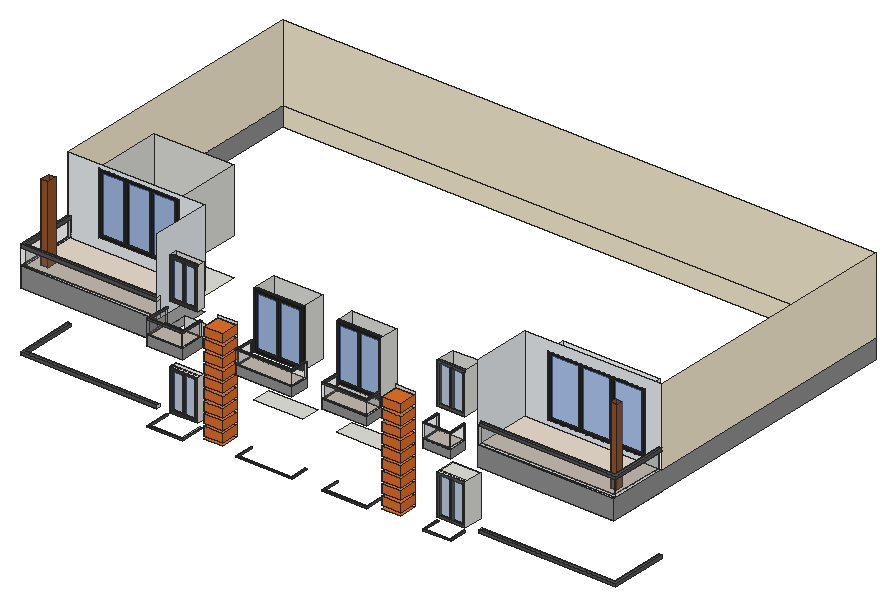
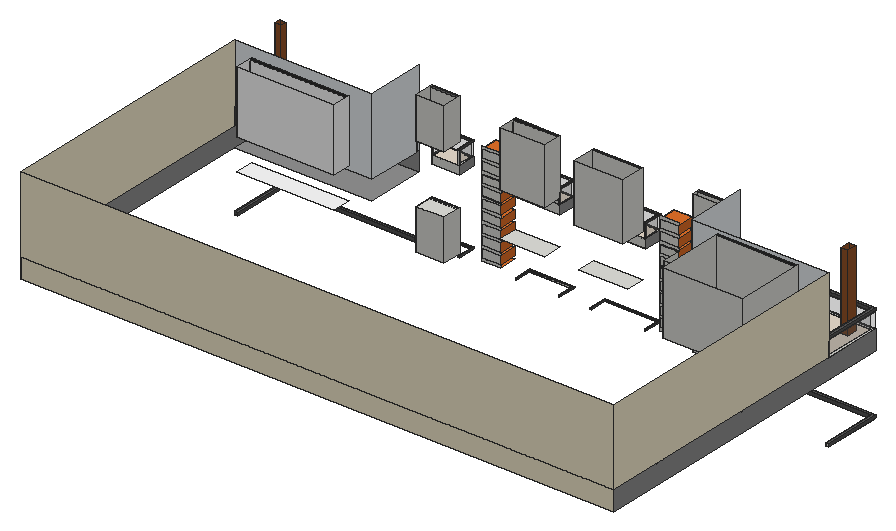
# SketchUp Ruby script. Lengths in inches.
U = 1.inch
M = Sketchup.active_model
def pt(a) = Geom::Point3d.new(a.map { |v| v * U })
def face(e, loops, mat)
  f = e.add_face(loops[0].map { |a| pt(a) })
  loops[1..].each { |l| e.add_face(l.map { |a| pt(a) }).erase! }
  f.material = f.back_material = mat if mat
  f
end
# faces: each face lists its corners as indices into pts; further lists are holes
def faces(e, pts, list, mat = nil) = list.each { |f| face(e, (f[0].is_a?(Array) ? f : [f]).map { |l| l.map { |i| pts[i] } }, mat) }
# xy, xz, yz: faces in a plane at the given z, y or x. An outline is a flat list of corners, or four numbers for a rectangle; further outlines are holes
def ring(l) = l.size == 4 ? [[l[0], l[1]], [l[2], l[1]], [l[2], l[3]], [l[0], l[3]]] : l.each_slice(2).to_a
def flat(e, list, mat, &to3) = list.each { |f| face(e, (f[0].is_a?(Array) ? f : [f]).map { |l| ring(l).map { |u, v| to3.(u, v) } }, mat) }
def xy(e, z, list, mat = nil) = flat(e, list, mat) { |x, y| [x, y, z] }
def xz(e, y, list, mat = nil) = flat(e, list, mat) { |x, z| [x, y, z] }
def yz(e, x, list, mat = nil) = flat(e, list, mat) { |y, z| [x, y, z] }
def lines(e, pts, list) = list.each { |a, b| e.add_line(pt(pts[a]), pt(pts[b])) }
# prism: a flat outline (further loops are holes) pulled along v
def prism(e, loops, v, mat = nil)
  f = face(e, loops, mat); d = Geom::Vector3d.new(v.map { |x| x * U })
  f.pushpull(f.normal.samedirection?(d) ? d.length : -d.length)
end
def box(e, o, s, mat = nil) = prism(e, [[o, [o[0] + s[0], o[1], o[2]], [o[0] + s[0], o[1] + s[1], o[2]], [o[0], o[1] + s[1], o[2]]]], [0, 0, s[2]], mat)
def at(x, y, z, deg = 0) = Geom::Transformation.translation(pt([x, y, z])) * Geom::Transformation.rotation(ORIGIN, Z_AXIS, deg.degrees)
def axes(o, x, y, z) = Geom::Transformation.new([*x, 0, *y, 0, *z, 0, *pt(o).to_a, 1])
def part(name) = M.definitions.add(name)
# library, detail: a bought-in or finely detailed component or shape, given as its bounding box
def library(name, o, s) = part(name).tap { |d| box(d.entities, o, s) }
def detail(e, o, s) = box(e.add_group.entities, o, s)
def put(e, d, t, mat = nil) = e.add_instance(d, t).tap { |i| i.material = mat if mat }
def group(e, t, mat = nil) = e.add_group.tap { |g| g.transformation = t; g.material = mat if mat }.entities
root = M.entities
M.materials.add("Generic").color = [146, 146, 146]
M.materials.add("Generic\#3").color = [226, 112, 41]
M.materials.add("Generic\#4").color = [237, 241, 244]
M.materials.add("Generic\#5").color = [249, 239, 211]
M.materials.add("Generic\#7").color = [232, 220, 205]
M.materials.add("[Color M00]").color = [255, 255, 255]
M.materials.add("[Color M06]").color = [86, 86, 86]
M.materials.add("[Color M07]").color = [58, 58, 58]
M.materials.add("[Color M08]").color = [30, 30, 30]
M.materials.add("[Translucent Glass Blue]").color = [98, 147, 234]
M.materials["[Translucent Glass Blue]"].alpha = 0.27
M.materials.add("[Translucent Glass Blue]1").color = [100, 149, 237]
M.materials["[Translucent Glass Blue]1"].alpha = 0.5
M.materials.add("[Translucent Glass Gray]").color = [119, 119, 119]
M.materials["[Translucent Glass Gray]"].alpha = 0.16
M.materials.add("[Wood Cherry Original]").color = [150, 85, 41]
M.materials.add("[Wood Cherry Original]1").color = [152, 86, 42]
c1 = part("Group\#1")
xy(c1.entities,0,[[0,0,60.75,6]],"[Color M07]")
xy(c1.entities,5.51,[[5.51,0,27.62,3],[33.13,0,55.24,3]],"[Color M07]")
xy(c1.entities,84.62,[[5.51,0,27.62,3],[33.13,0,55.24,3]])
xy(c1.entities,90.125,[[0,0,60.75,6]],"[Color M07]")
xz(c1.entities,0,[[[0,0,60.75,90.125],[5.51,5.51,27.62,84.62],[33.13,5.51,55.24,84.62]]],"[Color M07]")
xz(c1.entities,3,[[5.51,5.51,27.62,84.62],[33.13,5.51,55.24,84.62]],"[Translucent Glass Blue]")
xz(c1.entities,6,[[0,0,60.75,90.125]])
yz(c1.entities,0,[[0,0,6,90.125]],"[Color M07]")
yz(c1.entities,5.51,[[0,5.51,3,84.62]],"[Color M07]")
yz(c1.entities,27.62,[[0,5.51,3,84.62]],"[Color M07]")
yz(c1.entities,33.13,[[0,5.51,3,84.62]],"[Color M07]")
yz(c1.entities,55.24,[[0,5.51,3,84.62]],"[Color M07]")
yz(c1.entities,60.75,[[0,0,6,90.125]],"[Color M07]")
c2 = part("Group\#2")
xy(c2.entities,0,[[0,0,60.75,6]],"[Color M06]")
xy(c2.entities,4.875,[[4.875,0,27.9375,3],[32.8125,0,55.875,3]],"[Color M06]")
xy(c2.entities,85.25,[[4.875,0,27.9375,3],[32.8125,0,55.875,3]],"[Color M06]")
xy(c2.entities,90.125,[[0,0,60.75,6]],"[Color M06]")
xz(c2.entities,0,[[[0,0,60.75,90.125],[4.875,4.875,27.9375,85.25],[32.8125,4.875,55.875,85.25]]],"[Color M06]")
xz(c2.entities,3,[[4.875,4.875,27.9375,85.25],[32.8125,4.875,55.875,85.25]],"[Translucent Glass Blue]")
xz(c2.entities,6,[[0,0,60.75,90.125]])
yz(c2.entities,0,[[0,0,6,90.125]],"[Color M06]")
yz(c2.entities,4.875,[[0,4.875,3,85.25]],"[Color M06]")
yz(c2.entities,27.9375,[[0,4.875,3,85.25]],"[Color M06]")
yz(c2.entities,32.8125,[[0,4.875,3,85.25]],"[Color M06]")
yz(c2.entities,55.875,[[0,4.875,3,85.25]],"[Color M06]")
yz(c2.entities,60.75,[[0,0,6,90.125]],"[Color M06]")
c3 = part("Group\#12")
xy(c3.entities,0,[[0,0,212.5625,7]],"[Color M08]")
xy(c3.entities,6.29,[[6.29,0,68.76,4],[75.05,0,137.52,4],[143.8,0,206.27,4]],"[Color M08]")
xy(c3.entities,131.21,[[6.29,0,68.76,4],[75.05,0,137.52,4],[143.8,0,206.27,4]],"[Color M08]")
xy(c3.entities,137.5,[[0,0,212.5625,7]],"[Color M08]")
xz(c3.entities,0,[[0,0,212.5625,6.29],[0,6.29,6.29,131.21],[68.76,6.29,75.05,131.21],[137.52,6.29,143.8,131.21],[206.27,6.29,212.5625,131.21],
  [0,131.21,212.5625,137.5]],"[Color M08]")
xz(c3.entities,4,[[6.29,6.29,68.76,131.21],[75.05,6.29,137.52,131.21],[143.8,6.29,206.27,131.21]],"[Translucent Glass Blue]1")
xz(c3.entities,7,[[0,0,212.5625,137.5]],"[Color M00]")
yz(c3.entities,0,[[0,0,7,137.5]],"[Color M08]")
yz(c3.entities,6.29,[[0,6.29,4,131.21]],"[Color M08]")
yz(c3.entities,68.76,[[0,6.29,4,131.21]],"[Color M08]")
yz(c3.entities,75.05,[[0,6.29,4,131.21]],"[Color M08]")
yz(c3.entities,137.52,[[0,6.29,4,131.21]],"[Color M08]")
yz(c3.entities,143.8,[[0,6.29,4,131.21]],"[Color M08]")
yz(c3.entities,206.27,[[0,6.29,4,131.21]],"[Color M08]")
yz(c3.entities,212.5625,[[0,0,7,137.5]],"[Color M08]")
c4 = part("Group\#10")
xy(c4.entities,0,[[0,0,98.1875,6]],"[Color M08]")
xy(c4.entities,5.79,[[5.79,0,46.2,3],[51.99,0,92.4,3]],"[Color M08]")
xy(c4.entities,117.02,[[5.79,0,46.2,3],[51.99,0,92.4,3]],"[Color M08]")
xy(c4.entities,122.8125,[[0,0,98.1875,6]],"[Color M08]")
xz(c4.entities,0,[[[0,0,98.1875,122.8125],[5.79,5.79,46.2,117.02],[51.99,5.79,92.4,117.02]]],"[Color M08]")
xz(c4.entities,3,[[5.79,5.79,46.2,117.02],[51.99,5.79,92.4,117.02]],"[Translucent Glass Blue]1")
xz(c4.entities,6,[[0,0,98.1875,122.8125]])
yz(c4.entities,0,[[0,0,6,122.8125]],"[Color M08]")
yz(c4.entities,5.79,[[0,5.79,3,117.02]],"[Color M08]")
yz(c4.entities,46.2,[[0,5.79,3,117.02]],"[Color M08]")
yz(c4.entities,51.99,[[0,5.79,3,117.02]],"[Color M08]")
yz(c4.entities,92.4,[[0,5.79,3,117.02]],"[Color M08]")
yz(c4.entities,98.1875,[[0,0,6,122.8125]],"[Color M08]")
c5 = part("Group\#11")
xy(c5.entities,0,[[0,0,175.8125,6]],"[Color M08]")
xy(c5.entities,7.33,[[7.33,0,56.16,3],[63.49,0,112.32,3],[119.65,0,168.48,3]],"[Color M08]")
xy(c5.entities,131.1,[[7.33,0,56.16,3],[63.49,0,112.32,3],[119.65,0,168.48,3]],"[Color M08]")
xy(c5.entities,138.4375,[[0,0,175.8125,6]],"[Color M08]")
xz(c5.entities,0,[[[0,0,175.8125,0,175.8125,131.1,168.48,131.1,168.48,7.33,119.65,7.33,119.65,131.1,175.8125,131.1,175.8125,138.4375,0,138.4375],[7.33,7.33,56.16,131.1],[63.49,7.33,112.32,131.1]]],"[Color M08]")
xz(c5.entities,3,[[7.33,7.33,56.16,131.1],[63.49,7.33,112.32,131.1],[119.65,7.33,168.48,131.1]],"[Translucent Glass Blue]1")
xz(c5.entities,6,[[0,0,175.8125,138.4375]])
yz(c5.entities,0,[[0,0,6,138.4375]],"[Color M08]")
yz(c5.entities,7.33,[[0,7.33,3,131.1]],"[Color M08]")
yz(c5.entities,56.16,[[0,7.33,3,131.1]],"[Color M08]")
yz(c5.entities,63.49,[[0,7.33,3,131.1]],"[Color M08]")
yz(c5.entities,112.32,[[0,7.33,3,131.1]],"[Color M08]")
yz(c5.entities,119.65,[[0,7.33,3,131.1]],"[Color M08]")
yz(c5.entities,168.48,[[0,7.33,3,131.1]],"[Color M08]")
yz(c5.entities,175.8125,[[0,0,6,138.4375]],"[Color M08]")
xy(root,1083.75,[[529.46,261.625,529.46,313.625,532.46,313.625,532.46,264.625,604.09,264.625,604.09,313.625,607.09,313.625,607.09,261.625],[714.9,273.75,838.15,276.75],[903.71,273.75,1001.9,276.75],[1125.09,273.75,1185.84,276.75],[714.9,276.75,717.9,313.625],
  [835.15,276.75,838.15,313.625],[903.71,276.75,906.71,313.625],[998.9,276.75,1001.9,313.625],[1125.09,276.75,1128.09,313.625],[1182.84,276.75,1185.84,313.625]])
xy(root,1086.5,[[529.46,261.625,607.09,261.625,607.09,313.625,604.09,313.625,604.09,264.625,532.46,264.625,532.46,313.625,529.46,313.625]],"[Color M06]")
xy(root,1086.75,[[714.9,273.75,838.15,273.75,838.15,313.625,835.15,313.625,835.15,276.75,717.9,276.75,717.9,313.625,714.9,313.625],[903.71,273.75,1001.9,273.75,1001.9,313.625,998.9,313.625,998.9,276.75,906.71,276.75,906.71,313.625,903.71,313.625],[1125.09,273.75,1185.84,273.75,1185.84,313.625,1182.84,313.625,1182.84,276.75,1128.09,276.75,1128.09,313.625,1125.09,313.625]],"[Color M06]")
xy(root,1089.75,[[209.5,313.625,509.5,320.625],[1213,318.25,1213,325.0625,1506,325.0625,1506,444.3125,1513,444.3125,1513,318.25],[209.5,320.625,216.5,444.3125]])
xy(root,1092.02,[[537.9,313.625,598.65,331.25],[1125.09,313.625,1185.84,356.375]])
xy(root,1094.87,[[643.375,273.75,685.0625,313.625],[1034.5,273.75,1076.1875,313.625]],"Generic\#3")
xy(root,1096.1875,[[1213,318.25,1513,318.25,1513,444.3125,1506,444.3125,1506,325.0625,1213,325.0625]],"[Color M06]")
xy(root,1096.75,[[209.5,313.625,509.5,313.625,509.5,320.625,216.5,320.625,216.5,444.3125,209.5,444.3125]],"[Color M06]")
xy(root,1101.37,[[643.375,273.75,685.0625,313.625],[1034.5,273.75,1076.1875,313.625]],"Generic\#3")
xy(root,1119.37,[[643.375,273.75,685.0625,313.625],[1034.5,273.75,1076.1875,313.625]],"Generic\#3")
xy(root,1125.87,[[643.375,273.75,685.0625,313.625],[1034.5,273.75,1076.1875,313.625]],"Generic\#3")
xy(root,1143.87,[[643.375,273.75,685.0625,313.625],[1034.5,273.75,1076.1875,313.625]],"Generic\#3")
xy(root,1150.37,[[643.375,273.75,685.0625,313.625],[1034.5,273.75,1076.1875,313.625]],"Generic\#3")
xy(root,1168.37,[[643.375,273.75,685.0625,313.625],[1034.5,273.75,1076.1875,313.625]],"Generic\#3")
xy(root,1174.87,[[643.375,273.75,685.0625,313.625],[1034.5,273.75,1076.1875,313.625]],"Generic\#3")
xy(root,1182.05,[[722.84,313.625,830.21,354]])
xy(root,1182.15,[[537.9,313.625,598.65,331.25],[903.71,313.625,1001.9,356.375],[1125.09,313.625,1185.84,356.375]])
xy(root,1192.87,[[643.375,273.75,685.0625,313.625],[1034.5,273.75,1076.1875,313.625]],"Generic\#3")
xy(root,1199.37,[[643.375,273.75,685.0625,313.625],[1034.5,273.75,1076.1875,313.625]],"Generic\#3")
xy(root,1202.07,[[276.39,444.3125,452.2,595.9375]])
xy(root,1204.51,[[1262.61,444.3125,1475.18,486.125]],"[Color M00]")
xy(root,1217.37,[[643.375,273.75,685.0625,313.625],[1034.5,273.75,1076.1875,313.625]],"Generic\#3")
xy(root,1221.75,[[[209.5,313.625,509.5,444.3125],[234.12,340.02,249.74,361.77]],[[1213,313.625,1513,444.3125],[1483.76,340.63,1497.19,353.98]]],"Generic")
xy(root,1223.87,[[643.375,273.75,685.0625,313.625],[1034.5,273.75,1076.1875,313.625]],"Generic\#3")
xy(root,1241.87,[[643.375,273.75,685.0625,313.625],[1034.5,273.75,1076.1875,313.625]],"Generic\#3")
xy(root,1243.125,[[529.46,261.625,607.09,313.625]],"Generic")
xy(root,1246.0625,[[714.9,273.75,838.15,313.625],[903.71,273.75,1001.9,313.625],[1125.09,273.75,1185.84,313.625]],"Generic")
xy(root,1248.37,[[643.375,273.75,685.0625,313.625],[1034.5,273.75,1076.1875,313.625]],"Generic\#3")
xy(root,1264.5,[[529.46,261.625,529.46,313.625,532.46,313.625,532.46,264.625,604.09,264.625,604.09,313.625,607.09,313.625,607.09,261.625],[714.9,273.75,838.15,276.75],[903.71,273.75,1001.9,276.75],[1125.09,273.75,1185.84,276.75],[714.9,276.75,717.9,313.625],
  [835.15,276.75,838.15,313.625],[903.71,276.75,906.71,313.625],[998.9,276.75,1001.9,313.625],[1125.09,276.75,1128.09,313.625],[1182.84,276.75,1185.84,313.625],
  [209.5,313.625,509.5,320.625],[1213,313.625,1513,317.375],[1213,317.375,1213,324.375,1506,324.375,1506,444.3125,1513,444.3125,1513,317.375],[209.5,320.625,216.5,444.3125],[234.12,340.02,249.74,361.77],
  [1483.76,340.63,1497.19,353.98]])
xy(root,1264.5,[[532.46,264.625,604.09,313.625],[717.9,276.75,835.15,313.625],[906.71,276.75,998.9,313.625],[1128.09,276.75,1182.84,313.625],[[216.5,320.625,509.5,444.3125],[234.12,340.02,249.74,361.77]],
  [[1213,324.375,1506,444.3125],[1483.76,340.63,1497.19,353.98]]],"Generic\#7")
xy(root,1266.37,[[643.375,273.75,685.0625,313.625],[1034.5,273.75,1076.1875,313.625]],"Generic\#3")
xy(root,1272.87,[[643.375,273.75,685.0625,313.625],[1034.5,273.75,1076.1875,313.625]],"Generic\#3")
xy(root,1273.69,[[1262.61,444.3125,1475.18,486.125]],"[Color M00]")
xy(root,1275.65,[[722.84,313.625,830.21,367.6875]])
xy(root,1278.71,[[903.71,313.625,1001.9,356.375]])
xy(root,1286.32,[[276.39,444.3125,452.2,595.9375]])
xy(root,1290.87,[[643.375,273.75,685.0625,313.625],[1034.5,273.75,1076.1875,313.625]],"Generic\#3")
xy(root,1294.5,[[529.46,261.625,529.46,313.625,532.46,313.625,532.46,264.625,604.09,264.625,604.09,313.625,607.09,313.625,607.09,261.625],[714.9,273.75,838.15,276.75],[903.71,273.75,1001.9,276.75],[1125.09,273.75,1185.84,276.75],[714.9,276.75,717.9,313.625],
  [835.15,276.75,838.15,313.625],[903.71,276.75,906.71,313.625],[998.9,276.75,1001.9,313.625],[1125.09,276.75,1128.09,313.625],[1182.84,276.75,1185.84,313.625]])
xy(root,1297.25,[[529.46,261.625,607.09,261.625,607.09,313.625,604.09,313.625,604.09,264.625,532.46,264.625,532.46,313.625,529.46,313.625]],"[Color M06]")
xy(root,1297.37,[[643.375,273.75,685.0625,313.625],[1034.5,273.75,1076.1875,313.625]],"Generic\#3")
xy(root,1297.5,[[714.9,273.75,838.15,273.75,838.15,313.625,835.15,313.625,835.15,276.75,717.9,276.75,717.9,313.625,714.9,313.625],[903.71,273.75,1001.9,273.75,1001.9,313.625,998.9,313.625,998.9,276.75,906.71,276.75,906.71,313.625,903.71,313.625],[1125.09,273.75,1185.84,273.75,1185.84,313.625,1182.84,313.625,1182.84,276.75,1128.09,276.75,1128.09,313.625,1125.09,313.625]],"[Color M06]")
xy(root,1300.5,[[209.5,313.625,509.5,320.625],[1213,317.375,1213,324.375,1506,324.375,1506,444.3125,1513,444.3125,1513,317.375],[209.5,320.625,216.5,444.3125]])
xy(root,1306.9375,[[1213,317.375,1513,317.375,1513,444.3125,1506,444.3125,1506,324.375,1213,324.375]],"[Color M06]")
xy(root,1307.5,[[209.5,313.625,509.5,313.625,509.5,320.625,216.5,320.625,216.5,444.3125,209.5,444.3125]],"[Color M06]")
xy(root,1311.4,[[537.9,313.625,598.65,331.25],[1125.09,313.625,1185.84,356.375]])
xy(root,1315.37,[[643.375,273.75,685.0625,313.625],[1034.5,273.75,1076.1875,313.625]],"Generic\#3")
xz(root,261.625,[[529.46,1243.125,607.09,1264.5]],"Generic")
xz(root,261.625,[[529.46,1083.75,607.09,1086.5],[529.46,1294.5,607.09,1297.25]],"[Color M06]")
xz(root,261.625,[[529.46,1264.5,607.09,1294.5]],"[Translucent Glass Gray]")
xz(root,264.625,[[532.46,1083.75,604.09,1086.5],[532.46,1294.5,604.09,1297.25]])
xz(root,264.625,[[532.46,1264.5,604.09,1294.5]],"[Translucent Glass Gray]")
xz(root,273.75,[[714.9,1246.0625,838.15,1264.5],[903.71,1246.0625,1001.9,1264.5],[1125.09,1246.0625,1185.84,1264.5]],"Generic")
xz(root,273.75,[[643.375,1101.37,685.0625,1119.37],[1034.5,1101.37,1076.1875,1119.37],[643.375,1125.87,685.0625,1143.87],[1034.5,1125.87,1076.1875,1143.87],[643.375,1150.37,685.0625,1168.37],
  [1034.5,1150.37,1076.1875,1168.37],[643.375,1174.87,685.0625,1192.87],[1034.5,1174.87,1076.1875,1192.87],[643.375,1199.37,685.0625,1217.37],[1034.5,1199.37,1076.1875,1217.37],
  [643.375,1223.87,685.0625,1241.87],[1034.5,1223.87,1076.1875,1241.87],[643.375,1248.37,685.0625,1266.37],[1034.5,1248.37,1076.1875,1266.37],[643.375,1272.87,685.0625,1290.87],
  [1034.5,1272.87,1076.1875,1290.87],[643.375,1297.37,685.0625,1315.37],[1034.5,1297.37,1076.1875,1315.37]],"Generic\#3")
xz(root,273.75,[[714.9,1083.75,838.15,1086.75],[903.71,1083.75,1001.9,1086.75],[1125.09,1083.75,1185.84,1086.75],[714.9,1294.5,838.15,1297.5],[903.71,1294.5,1001.9,1297.5],
  [1125.09,1294.5,1185.84,1297.5]],"[Color M06]")
xz(root,273.75,[[714.9,1264.5,838.15,1294.5],[903.71,1264.5,1001.9,1294.5],[1125.09,1264.5,1185.84,1294.5]],"[Translucent Glass Gray]")
xz(root,276.75,[[717.9,1083.75,835.15,1086.75],[906.71,1083.75,998.9,1086.75],[1128.09,1083.75,1182.84,1086.75],[717.9,1294.5,835.15,1297.5],[906.71,1294.5,998.9,1297.5]])
xz(root,276.75,[[1128.09,1294.5,1182.84,1297.5]],"[Color M06]")
xz(root,276.75,[[717.9,1264.5,835.15,1294.5],[906.71,1264.5,998.9,1294.5],[1128.09,1264.5,1182.84,1294.5]],"[Translucent Glass Gray]")
xz(root,313.625,[[714.9,1083.75,717.9,1086.75],[835.15,1083.75,838.15,1086.75],[903.71,1083.75,906.71,1086.75],[998.9,1083.75,1001.9,1086.75],[1125.09,1083.75,1128.09,1086.75],
  [1182.84,1083.75,1185.84,1086.75],[643.375,1094.87,685.0625,1101.37],[1034.5,1094.87,1076.1875,1101.37],[643.375,1101.37,685.0625,1119.37],[1034.5,1101.37,1076.1875,1119.37],
  [643.375,1119.37,685.0625,1125.87],[1034.5,1119.37,1076.1875,1125.87],[643.375,1125.87,685.0625,1143.87],[1034.5,1125.87,1076.1875,1143.87],[643.375,1143.87,685.0625,1150.37],
  [1034.5,1143.87,1076.1875,1150.37],[643.375,1150.37,685.0625,1168.37],[1034.5,1150.37,1076.1875,1168.37],[643.375,1168.37,685.0625,1174.87],[1034.5,1168.37,1076.1875,1174.87],
  [643.375,1174.87,685.0625,1192.87],[1034.5,1174.87,1076.1875,1192.87],[643.375,1192.87,685.0625,1199.37],[1034.5,1192.87,1076.1875,1199.37],[643.375,1199.37,685.0625,1217.37],
  [1034.5,1199.37,1076.1875,1217.37],[643.375,1217.37,685.0625,1221.75],[1034.5,1217.37,1076.1875,1221.75],[643.375,1221.75,685.0625,1223.87],[1034.5,1221.75,1076.1875,1223.87],
  [643.375,1223.87,685.0625,1241.87],[1034.5,1223.87,1076.1875,1241.87],[643.375,1241.87,685.0625,1248.37],[1034.5,1241.87,1076.1875,1248.37],[529.46,1243.125,607.09,1264.5],
  [714.9,1246.0625,838.15,1264.5],[903.71,1246.0625,1001.9,1264.5],[1125.09,1246.0625,1185.84,1264.5],[643.375,1248.37,685.0625,1264.5],[1034.5,1248.37,1076.1875,1264.5],
  [643.375,1264.5,685.0625,1266.37],[714.9,1264.5,717.9,1294.5],[835.15,1264.5,838.15,1294.5],[903.71,1264.5,906.71,1278.71],[906.71,1264.5,998.9,1278.71],
  [998.9,1264.5,1001.9,1278.71],[1034.5,1264.5,1076.1875,1266.37],[1125.09,1264.5,1128.09,1294.5],[1182.84,1264.5,1185.84,1294.5],[643.375,1266.37,685.0625,1272.87],
  [1034.5,1266.37,1076.1875,1272.87],[643.375,1272.87,685.0625,1290.87],[1034.5,1272.87,1076.1875,1290.87],[903.71,1278.71,906.71,1294.5],[998.9,1278.71,1001.9,1294.5],
  [643.375,1290.87,685.0625,1297.37],[1034.5,1290.87,1076.1875,1297.37],[714.9,1294.5,717.9,1297.5],[835.15,1294.5,838.15,1297.5],[903.71,1294.5,906.71,1297.5],
  [998.9,1294.5,1001.9,1297.5],[1125.09,1294.5,1128.09,1297.5],[1182.84,1294.5,1185.84,1297.5],[643.375,1297.37,685.0625,1315.37],[1034.5,1297.37,1076.1875,1315.37],
  [643.375,1315.37,685.0625,1321.87],[1034.5,1315.37,1076.1875,1321.87]])
xz(root,313.625,[[209.5,1221.75,509.5,1264.5],[1213,1221.75,1513,1264.5]],"Generic")
xz(root,313.625,[[209.5,1089.75,509.5,1096.75],[209.5,1300.5,509.5,1307.5]],"[Color M06]")
xz(root,313.625,[[209.5,1264.5,509.5,1300.5]],"[Translucent Glass Gray]")
xz(root,317.375,[[1213,1300.5,1513,1306.9375]],"[Color M06]")
xz(root,317.375,[[1213,1264.5,1513,1300.5]],"[Translucent Glass Gray]")
xz(root,318.25,[[1213,1089.75,1513,1096.1875]],"[Color M06]")
xz(root,320.625,[[216.5,1089.75,509.5,1096.75],[216.5,1300.5,509.5,1307.5]],"[Color M06]")
xz(root,320.625,[[216.5,1264.5,509.5,1300.5]],"[Translucent Glass Gray]")
xz(root,324.375,[[1213,1300.5,1506,1306.9375]],"[Color M06]")
xz(root,324.375,[[1213,1264.5,1506,1300.5]],"[Translucent Glass Gray]")
xz(root,325.0625,[[1213,1089.75,1506,1096.1875]],"[Color M06]")
xz(root,331.25,[[537.9,1092.02,598.65,1182.15],[537.9,1311.4,598.65,1401.52]])
xz(root,340.02,[[234.12,1264.5,249.74,1432.5]],"[Wood Cherry Original]1")
xz(root,340.63,[[1483.76,1264.5,1497.19,1432.5]],"[Wood Cherry Original]")
xz(root,353.875,[[537.9,1221.75,643.375,1264.5]])
xz(root,353.98,[[1483.76,1264.5,1497.19,1432.5]],"[Wood Cherry Original]")
xz(root,356.375,[[1125.09,1092.02,1185.84,1182.15],[903.71,1278.71,1001.9,1401.52],[1125.09,1311.4,1185.84,1401.52]])
xz(root,361.77,[[234.12,1264.5,249.74,1432.5]],"[Wood Cherry Original]1")
xz(root,367.6875,[[722.84,1275.65,830.21,1401.52]])
xz(root,444.3125,[[209.5,1089.75,216.5,1096.75],[209.5,1264.5,216.5,1300.5],[209.5,1300.5,216.5,1307.5]])
xz(root,444.3125,[[[216.5,1264.5,509.5,1264.5,509.5,1432.5,209.5,1432.5,209.5,1307.5,216.5,1307.5],[276.39,1286.32,452.2,1424.76]],[[1213,1264.5,1506,1264.5,1506,1306.9375,1513,1306.9375,1513,1432.5,1213,1432.5],[1262.61,1273.69,1475.18,1411.19]]],"Generic\#4")
xz(root,486.125,[[1262.61,1273.69,1475.18,1411.19]],"[Color M00]")
xz(root,595.9375,[[276.39,1286.32,452.2,1424.76]])
xz(root,1033.625,[[209.5,1221.75,1513,1264.5],[209.5,1264.5,1513,1432.5]],"Generic\#5")
yz(root,209.5,[[313.625,1221.75,1033.625,1264.5]],"Generic")
yz(root,209.5,[[444.3125,1264.5,1033.625,1432.5]],"Generic\#5")
yz(root,209.5,[[313.625,1089.75,444.3125,1096.75],[313.625,1300.5,444.3125,1307.5]],"[Color M06]")
yz(root,209.5,[[313.625,1264.5,444.3125,1300.5]],"[Translucent Glass Gray]")
yz(root,216.5,[[320.625,1089.75,444.3125,1096.75],[320.625,1300.5,444.3125,1307.5]],"[Color M06]")
yz(root,216.5,[[320.625,1264.5,444.3125,1300.5]],"[Translucent Glass Gray]")
yz(root,234.12,[[340.02,1264.5,361.77,1432.5]],"[Wood Cherry Original]1")
yz(root,249.74,[[340.02,1264.5,361.77,1432.5]],"[Wood Cherry Original]1")
yz(root,276.39,[[444.3125,1286.32,595.9375,1424.76]])
yz(root,452.2,[[444.3125,1286.32,595.9375,1424.76]])
yz(root,509.5,[[313.625,1089.75,320.625,1096.75],[313.625,1264.5,320.625,1300.5],[313.625,1300.5,320.625,1307.5]])
yz(root,509.5,[[320.625,1264.5,320.625,1307.5,313.625,1307.5,313.625,1432.5,444.3125,1432.5,444.3125,1264.5]],"Generic\#4")
yz(root,529.46,[[261.625,1243.125,313.625,1264.5]],"Generic")
yz(root,529.46,[[261.625,1083.75,313.625,1086.5],[261.625,1294.5,313.625,1297.25]],"[Color M06]")
yz(root,529.46,[[261.625,1264.5,313.625,1294.5]],"[Translucent Glass Gray]")
yz(root,532.46,[[264.625,1083.75,313.625,1086.5],[264.625,1294.5,313.625,1297.25]],"[Color M06]")
yz(root,532.46,[[264.625,1264.5,313.625,1294.5]],"[Translucent Glass Gray]")
yz(root,537.9,[[313.625,1092.02,331.25,1182.15],[313.625,1311.4,331.25,1401.52]])
yz(root,598.65,[[313.625,1092.02,331.25,1182.15],[313.625,1311.4,331.25,1401.52]])
yz(root,604.09,[[264.625,1083.75,313.625,1086.5]])
yz(root,604.09,[[264.625,1294.5,313.625,1297.25]],"[Color M06]")
yz(root,604.09,[[264.625,1264.5,313.625,1294.5]],"[Translucent Glass Gray]")
yz(root,607.09,[[261.625,1243.125,313.625,1264.5]],"Generic")
yz(root,607.09,[[261.625,1083.75,313.625,1086.5],[261.625,1294.5,313.625,1297.25]],"[Color M06]")
yz(root,607.09,[[261.625,1264.5,313.625,1294.5]],"[Translucent Glass Gray]")
yz(root,643.375,[[313.625,1221.75,353.875,1264.5]])
yz(root,643.375,[[273.75,1101.37,313.625,1119.37],[273.75,1125.87,313.625,1143.87],[273.75,1150.37,313.625,1168.37],[273.75,1174.87,313.625,1192.87],[273.75,1199.37,313.625,1217.37],
  [273.75,1223.87,313.625,1241.87],[273.75,1248.37,313.625,1266.37],[273.75,1272.87,313.625,1290.87],[273.75,1297.37,313.625,1315.37]],"Generic\#3")
yz(root,685.0625,[[273.75,1101.37,313.625,1119.37],[273.75,1125.87,313.625,1143.87],[273.75,1150.37,313.625,1168.37],[273.75,1174.87,313.625,1192.87],[273.75,1199.37,313.625,1217.37],
  [273.75,1223.87,313.625,1241.87],[273.75,1248.37,313.625,1266.37],[273.75,1272.87,313.625,1290.87],[273.75,1297.37,313.625,1315.37]],"Generic\#3")
yz(root,714.9,[[273.75,1246.0625,313.625,1264.5]],"Generic")
yz(root,714.9,[[273.75,1083.75,313.625,1086.75],[273.75,1294.5,313.625,1297.5]],"[Color M06]")
yz(root,714.9,[[273.75,1264.5,313.625,1294.5]],"[Translucent Glass Gray]")
yz(root,717.9,[[276.75,1083.75,313.625,1086.75],[276.75,1294.5,313.625,1297.5]],"[Color M06]")
yz(root,717.9,[[276.75,1264.5,313.625,1294.5]],"[Translucent Glass Gray]")
yz(root,722.84,[[313.625,1275.65,367.6875,1401.52]])
yz(root,830.21,[[313.625,1275.65,367.6875,1401.52]])
yz(root,835.15,[[276.75,1083.75,313.625,1086.75],[276.75,1294.5,313.625,1297.5]],"[Color M06]")
yz(root,835.15,[[276.75,1264.5,313.625,1294.5]],"[Translucent Glass Gray]")
yz(root,838.15,[[273.75,1246.0625,313.625,1264.5]],"Generic")
yz(root,838.15,[[273.75,1083.75,313.625,1086.75],[273.75,1294.5,313.625,1297.5]],"[Color M06]")
yz(root,838.15,[[273.75,1264.5,313.625,1294.5]],"[Translucent Glass Gray]")
yz(root,903.71,[[313.625,1278.71,356.375,1401.52]])
yz(root,903.71,[[273.75,1246.0625,313.625,1264.5]],"Generic")
yz(root,903.71,[[273.75,1083.75,313.625,1086.75],[273.75,1294.5,313.625,1297.5]],"[Color M06]")
yz(root,903.71,[[273.75,1264.5,313.625,1294.5]],"[Translucent Glass Gray]")
yz(root,906.71,[[276.75,1083.75,313.625,1086.75],[276.75,1294.5,313.625,1297.5]],"[Color M06]")
yz(root,906.71,[[276.75,1264.5,313.625,1294.5]],"[Translucent Glass Gray]")
yz(root,998.9,[[276.75,1083.75,313.625,1086.75],[276.75,1294.5,313.625,1297.5]],"[Color M06]")
yz(root,998.9,[[276.75,1264.5,313.625,1294.5]],"[Translucent Glass Gray]")
yz(root,1001.9,[[313.625,1278.71,356.375,1401.52]])
yz(root,1001.9,[[273.75,1246.0625,313.625,1264.5]],"Generic")
yz(root,1001.9,[[273.75,1083.75,313.625,1086.75],[273.75,1294.5,313.625,1297.5]],"[Color M06]")
yz(root,1001.9,[[273.75,1264.5,313.625,1294.5]],"[Translucent Glass Gray]")
yz(root,1034.5,[[273.75,1101.37,313.625,1119.37],[273.75,1125.87,313.625,1143.87],[273.75,1150.37,313.625,1168.37],[273.75,1174.87,313.625,1192.87],[273.75,1199.37,313.625,1217.37],
  [273.75,1223.87,313.625,1241.87],[273.75,1248.37,313.625,1266.37],[273.75,1272.87,313.625,1290.87],[273.75,1297.37,313.625,1315.37]],"Generic\#3")
yz(root,1076.1875,[[273.75,1101.37,313.625,1119.37],[273.75,1125.87,313.625,1143.87],[273.75,1150.37,313.625,1168.37],[273.75,1174.87,313.625,1192.87],[273.75,1199.37,313.625,1217.37],
  [273.75,1223.87,313.625,1241.87],[273.75,1248.37,313.625,1266.37],[273.75,1272.87,313.625,1290.87],[273.75,1297.37,313.625,1315.37]],"Generic\#3")
yz(root,1125.09,[[313.625,1092.02,356.375,1182.15],[313.625,1311.4,356.375,1401.52]])
yz(root,1125.09,[[273.75,1246.0625,313.625,1264.5]],"Generic")
yz(root,1125.09,[[273.75,1083.75,313.625,1086.75],[273.75,1294.5,313.625,1297.5]],"[Color M06]")
yz(root,1125.09,[[273.75,1264.5,313.625,1294.5]],"[Translucent Glass Gray]")
yz(root,1128.09,[[276.75,1083.75,313.625,1086.75],[276.75,1294.5,313.625,1297.5]],"[Color M06]")
yz(root,1128.09,[[276.75,1264.5,313.625,1294.5]],"[Translucent Glass Gray]")
yz(root,1182.84,[[276.75,1083.75,313.625,1086.75],[276.75,1294.5,313.625,1297.5]],"[Color M06]")
yz(root,1182.84,[[276.75,1264.5,313.625,1294.5]],"[Translucent Glass Gray]")
yz(root,1185.84,[[313.625,1092.02,356.375,1182.15],[313.625,1311.4,356.375,1401.52]])
yz(root,1185.84,[[273.75,1246.0625,313.625,1264.5]],"Generic")
yz(root,1185.84,[[273.75,1083.75,313.625,1086.75],[273.75,1294.5,313.625,1297.5]],"[Color M06]")
yz(root,1185.84,[[273.75,1264.5,313.625,1294.5]],"[Translucent Glass Gray]")
yz(root,1213,[[318.25,1089.75,325.0625,1096.1875],[317.375,1264.5,324.375,1300.5],[317.375,1300.5,324.375,1306.9375]])
yz(root,1213,[[313.625,1264.5,317.375,1264.5,317.375,1306.9375,324.375,1306.9375,324.375,1264.5,444.3125,1264.5,444.3125,1432.5,313.625,1432.5]],"Generic\#4")
yz(root,1262.61,[[444.3125,1273.69,486.125,1411.19]],"[Color M00]")
yz(root,1475.18,[[444.3125,1273.69,486.125,1411.19]],"[Color M00]")
yz(root,1483.76,[[340.63,1264.5,353.98,1432.5]],"[Wood Cherry Original]")
yz(root,1497.19,[[340.63,1264.5,353.98,1432.5]],"[Wood Cherry Original]")
yz(root,1506,[[324.375,1300.5,444.3125,1306.9375]])
yz(root,1506,[[325.0625,1089.75,444.3125,1096.1875]],"[Color M06]")
yz(root,1506,[[324.375,1264.5,444.3125,1300.5]],"[Translucent Glass Gray]")
yz(root,1513,[[313.625,1221.75,1033.625,1264.5]],"Generic")
yz(root,1513,[[444.3125,1264.5,1033.625,1432.5]],"Generic\#5")
yz(root,1513,[[318.25,1089.75,444.3125,1096.1875],[317.375,1300.5,444.3125,1306.9375]],"[Color M06]")
yz(root,1513,[[317.375,1264.5,444.3125,1300.5]],"[Translucent Glass Gray]")
p = [[537.9,313.625,1264.5],[537.9,353.875,1264.5],[537.9,313.625,1221.75],[537.9,353.875,1221.75]]
lines(root,p,[[0,1],[2,3]])
put(root,c1,at(537.9,313.625,1092.02))
put(root,c2,at(1125.09,313.625,1092.02))
put(root,c3,at(1262.61,444.3125,1273.69))
g1 = group(root,at(722.84,313.625,1275.65))
xy(g1,0,[[0,0,107.375,6]],"[Color M08]")
xy(g1,6.51,[[6.51,0,50.43,3],[56.94,0,100.87,3]],"[Color M08]")
xy(g1,119.37,[[6.51,0,50.43,3],[56.94,0,100.87,3]],"[Color M08]")
xy(g1,125.875,[[0,0,107.375,6]],"[Color M08]")
xz(g1,0,[[[0,0,107.375,125.875],[6.51,6.51,50.43,119.37],[56.94,6.51,100.87,119.37]]],"[Color M08]")
xz(g1,3,[[6.51,6.51,50.43,119.37],[56.94,6.51,100.87,119.37]],"[Translucent Glass Blue]1")
xz(g1,6,[[0,0,107.375,125.875]])
yz(g1,0,[[0,0,6,125.875]],"[Color M08]")
yz(g1,6.51,[[0,6.51,3,119.37]],"[Color M08]")
yz(g1,50.43,[[0,6.51,3,119.37]],"[Color M08]")
yz(g1,56.94,[[0,6.51,3,119.37]],"[Color M08]")
yz(g1,100.87,[[0,6.51,3,119.37]],"[Color M08]")
yz(g1,107.375,[[0,0,6,125.875]],"[Color M08]")
put(root,c4,at(903.71,313.625,1278.71))
put(root,c5,at(276.39,444.3125,1286.32))
put(root,c1,at(537.9,313.625,1311.4))
put(root,c2,at(1125.09,313.625,1311.4))
